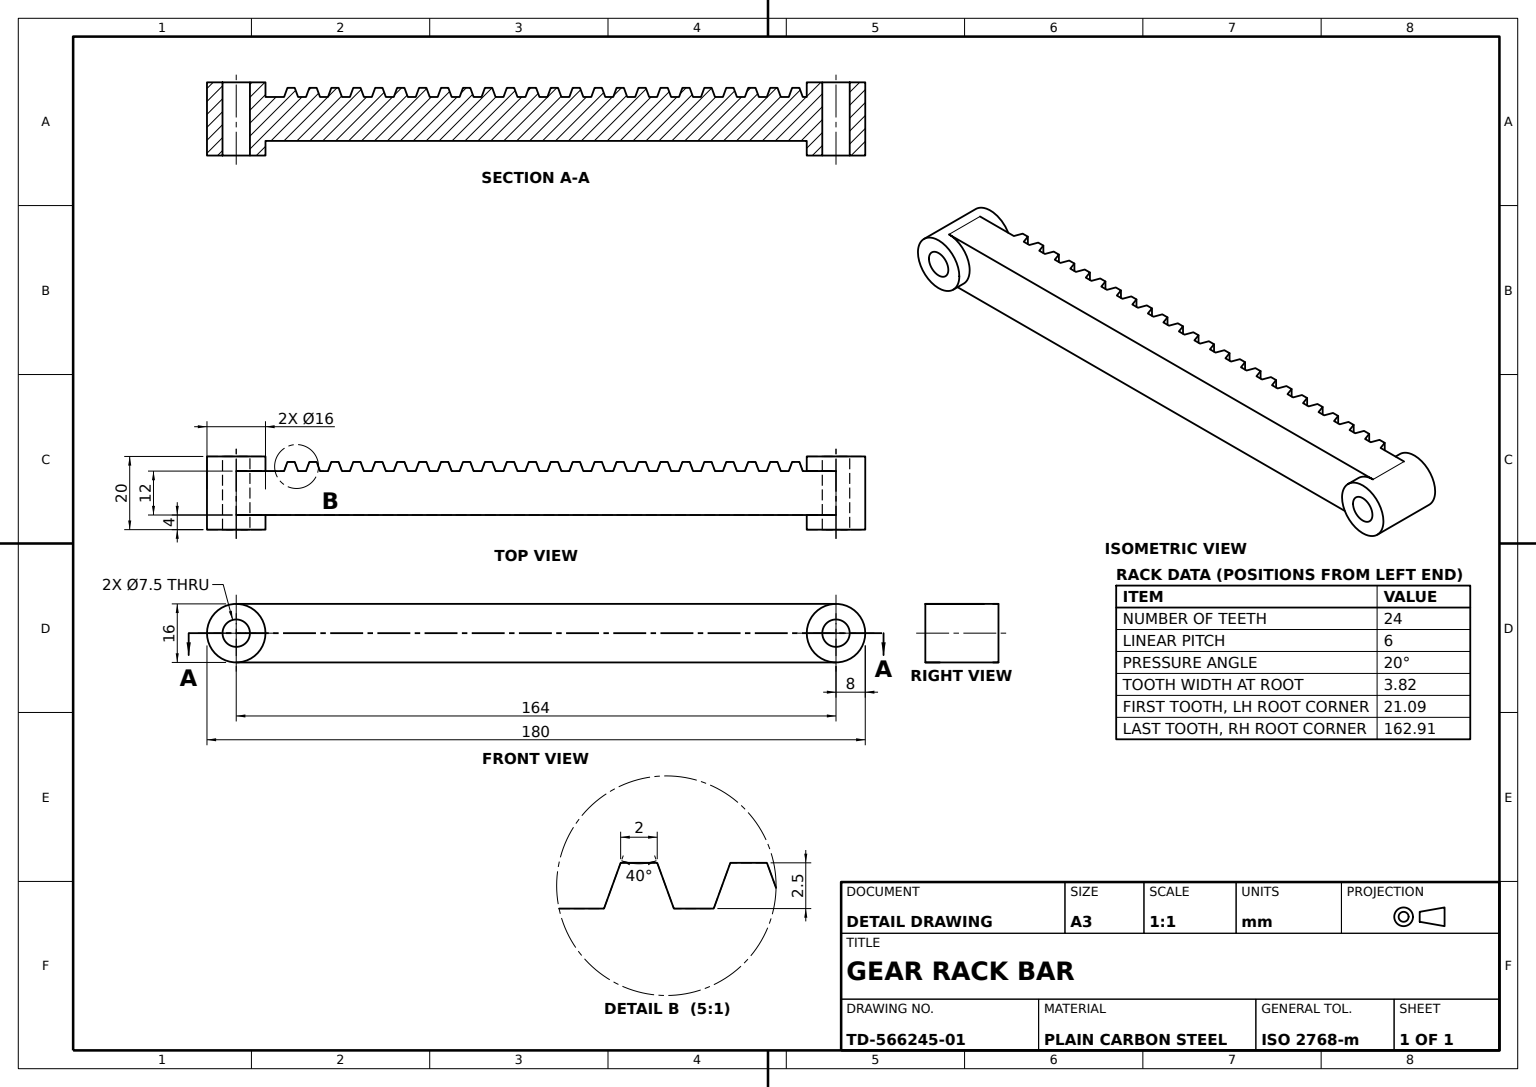
solid
v1 (10,0,8)
v2 (10,0,-8)
e1 v1 v2 CIRCLE(AX(P(10,0,0),D(1,0,0),D(0,0,-1)),8)
v3 (6,0,8)
e2 v1 v3 LINE
v4 (6,-8,0)
e3 v4 v3 CIRCLE(AX(P(6,0,0),D(-1,0,0),D(0,0,-1)),8)
v5 (-6,-8,0)
e4 v4 v5 LINE
v6 (-6,0,8)
e5 v5 v6 CIRCLE(AX(P(-6,0,0),D(-1,0,0),D(0,0,-1)),8)
v7 (-10,0,8)
e6 v6 v7 LINE
v8 (-10,0,-8)
e7 v7 v8 CIRCLE(AX(P(-10,0,0),D(1,0,0),D(0,0,-1)),8)
e8 v2 v8 LINE
face CYL(AX(P(10,0,0),D(-1,0,0),D(0,0,1)),8) [-e1 e2 -e3 e4 e5 e6 e7 -e8]
v9 (-8.5,8,100)
v10 (-8.5,8,102)
e9 v9 v10 LINE
v11 (-8.5,-8,100)
e10 v9 v11 LINE
v12 (-8.5,-8,102)
e11 v11 v12 LINE
e12 v10 v12 LINE
face PLANE(AX(P(-8.5,8,100),D(1,0,0),D(0,0,-1))) rev [-e9 e10 e11 -e12]
v13 (-6,-8,15.090074)
v14 (-6,-8,12.909926)
e13 v13 v14 LINE
v15 (-6,8,15.090074)
e14 v15 v13 LINE
v16 (-6,8,12.909926)
e15 v16 v15 LINE
e16 v14 v16 LINE
face PLANE(AX(P(-6,0,164),D(1,0,0),D(0,0,-1))) rev [-e13 -e14 -e15 -e16]
v17 (10,0,3.75)
v18 (-10,0,3.75)
e17 v17 v18 LINE
v19 (10,0,-3.75)
e18 v17 v19 CIRCLE(AX(P(10,0,0),D(1,0,0),D(0,0,-1)),3.75)
v20 (-10,0,-3.75)
e19 v19 v20 LINE
e20 v18 v20 CIRCLE(AX(P(-10,0,0),D(1,0,0),D(0,0,-1)),3.75)
face CYL(AX(P(10,0,0),D(-1,0,0),D(0,0,1)),3.75) rev [-e17 e18 e19 -e20]
v21 (-8.5,8,138)
v22 (-6,8,138.909926)
e21 v21 v22 LINE
v23 (-8.5,-8,138)
e22 v21 v23 LINE
v24 (-6,-8,138.909926)
e23 v23 v24 LINE
e24 v24 v22 LINE
face PLANE(AX(P(-8.5,8,138),D(0.342020143,0,-0.939692621),D(-0.939692621,0,-0.342020143))) rev [-e21 e22 e23 e24]
v25 (-6,8,27.090074)
v26 (-8.5,8,28)
e25 v25 v26 LINE
v27 (-6,-8,27.090074)
e26 v25 v27 LINE
v28 (-8.5,-8,28)
e27 v27 v28 LINE
e28 v26 v28 LINE
face PLANE(AX(P(-8.5,8,28),D(0.342020143,0,0.939692621),D(0.939692621,0,-0.342020143))) rev [-e25 e26 e27 -e28]
v29 (-8.5,8,36)
v30 (-6,8,36.909926)
e29 v29 v30 LINE
v31 (-8.5,-8,36)
e30 v29 v31 LINE
v32 (-6,-8,36.909926)
e31 v31 v32 LINE
e32 v32 v30 LINE
face PLANE(AX(P(-8.5,8,36),D(0.342020143,0,-0.939692621),D(-0.939692621,0,-0.342020143))) rev [-e29 e30 e31 e32]
v33 (-6,0,156)
v34 (-10,0,156)
e33 v33 v34 LINE
v35 (-10,0,172)
e34 v34 v35 CIRCLE(AX(P(-10,0,164),D(1,0,0),D(0,0,-1)),8)
v36 (10,0,172)
e35 v36 v35 LINE
v37 (10,0,156)
e36 v37 v36 CIRCLE(AX(P(10,0,164),D(1,0,0),D(0,0,-1)),8)
v38 (6,0,156)
e37 v37 v38 LINE
v39 (6,8,164)
e38 v39 v38 CIRCLE(AX(P(6,0,164),D(-1,0,0),D(0,0,-1)),8)
v40 (-6,8,164)
e39 v39 v40 LINE
e40 v40 v33 CIRCLE(AX(P(-6,0,164),D(-1,0,0),D(0,0,-1)),8)
face CYL(AX(P(10,0,164),D(-1,0,0),D(0,0,1)),8) [e33 e34 -e35 -e36 e37 -e38 e39 e40]
v41 (-8.5,8,124)
v42 (-8.5,8,126)
e41 v41 v42 LINE
v43 (-6,8,126.909926)
e42 v42 v43 LINE
v44 (-6,8,129.090074)
e43 v43 v44 LINE
v45 (-8.5,8,130)
e44 v44 v45 LINE
v46 (-8.5,8,132)
e45 v45 v46 LINE
v47 (-6,8,132.909926)
e46 v46 v47 LINE
v48 (-6,8,135.090074)
e47 v47 v48 LINE
v49 (-8.5,8,136)
e48 v48 v49 LINE
e49 v49 v21 LINE
v50 (-6,8,141.090074)
e50 v22 v50 LINE
v51 (-8.5,8,142)
e51 v50 v51 LINE
v52 (-8.5,8,144)
e52 v51 v52 LINE
v53 (-6,8,144.909926)
e53 v52 v53 LINE
v54 (-6,8,147.090074)
e54 v53 v54 LINE
v55 (-8.5,8,148)
e55 v54 v55 LINE
v56 (-8.5,8,150)
e56 v55 v56 LINE
v57 (-6,8,150.909926)
e57 v56 v57 LINE
e58 v57 v40 LINE
v58 (6,8,0)
e59 v58 v39 LINE
v59 (-6,8,0)
e60 v58 v59 LINE
v60 (-6,8,9.090074)
e61 v59 v60 LINE
v61 (-8.5,8,10)
e62 v60 v61 LINE
v62 (-8.5,8,12)
e63 v61 v62 LINE
e64 v62 v16 LINE
v63 (-8.5,8,16)
e65 v15 v63 LINE
v64 (-8.5,8,18)
e66 v63 v64 LINE
v65 (-6,8,18.909926)
e67 v64 v65 LINE
v66 (-6,8,21.090074)
e68 v65 v66 LINE
v67 (-8.5,8,22)
e69 v66 v67 LINE
v68 (-8.5,8,24)
e70 v67 v68 LINE
v69 (-6,8,24.909926)
e71 v68 v69 LINE
e72 v69 v25 LINE
v70 (-8.5,8,30)
e73 v26 v70 LINE
v71 (-6,8,30.909926)
e74 v70 v71 LINE
v72 (-6,8,33.090074)
e75 v71 v72 LINE
v73 (-8.5,8,34)
e76 v72 v73 LINE
e77 v73 v29 LINE
v74 (-6,8,39.090074)
e78 v30 v74 LINE
v75 (-8.5,8,40)
e79 v74 v75 LINE
v76 (-8.5,8,42)
e80 v75 v76 LINE
v77 (-6,8,42.909926)
e81 v76 v77 LINE
v78 (-6,8,45.090074)
e82 v77 v78 LINE
v79 (-8.5,8,46)
e83 v78 v79 LINE
v80 (-8.5,8,48)
e84 v79 v80 LINE
v81 (-6,8,48.909926)
e85 v80 v81 LINE
v82 (-6,8,51.090074)
e86 v81 v82 LINE
v83 (-8.5,8,52)
e87 v82 v83 LINE
v84 (-8.5,8,54)
e88 v83 v84 LINE
v85 (-6,8,54.909926)
e89 v84 v85 LINE
v86 (-6,8,57.090074)
e90 v85 v86 LINE
v87 (-8.5,8,58)
e91 v86 v87 LINE
v88 (-8.5,8,60)
e92 v87 v88 LINE
v89 (-6,8,60.909926)
e93 v88 v89 LINE
v90 (-6,8,63.090074)
e94 v89 v90 LINE
v91 (-8.5,8,64)
e95 v90 v91 LINE
v92 (-8.5,8,66)
e96 v91 v92 LINE
v93 (-6,8,66.909926)
e97 v92 v93 LINE
v94 (-6,8,69.090074)
e98 v93 v94 LINE
v95 (-8.5,8,70)
e99 v94 v95 LINE
v96 (-8.5,8,72)
e100 v95 v96 LINE
v97 (-6,8,72.909926)
e101 v96 v97 LINE
v98 (-6,8,75.090074)
e102 v97 v98 LINE
v99 (-8.5,8,76)
e103 v98 v99 LINE
v100 (-8.5,8,78)
e104 v99 v100 LINE
v101 (-6,8,78.909926)
e105 v100 v101 LINE
v102 (-6,8,81.090074)
e106 v101 v102 LINE
v103 (-8.5,8,82)
e107 v102 v103 LINE
v104 (-8.5,8,84)
e108 v103 v104 LINE
v105 (-6,8,84.909926)
e109 v104 v105 LINE
v106 (-6,8,87.090074)
e110 v105 v106 LINE
v107 (-8.5,8,88)
e111 v106 v107 LINE
v108 (-8.5,8,90)
e112 v107 v108 LINE
v109 (-6,8,90.909926)
e113 v108 v109 LINE
v110 (-6,8,93.090074)
e114 v109 v110 LINE
v111 (-8.5,8,94)
e115 v110 v111 LINE
v112 (-8.5,8,96)
e116 v111 v112 LINE
v113 (-6,8,96.909926)
e117 v112 v113 LINE
v114 (-6,8,99.090074)
e118 v113 v114 LINE
e119 v114 v9 LINE
v115 (-6,8,102.909926)
e120 v10 v115 LINE
v116 (-6,8,105.090074)
e121 v115 v116 LINE
v117 (-8.5,8,106)
e122 v116 v117 LINE
v118 (-8.5,8,108)
e123 v117 v118 LINE
v119 (-6,8,108.909926)
e124 v118 v119 LINE
v120 (-6,8,111.090074)
e125 v119 v120 LINE
v121 (-8.5,8,112)
e126 v120 v121 LINE
v122 (-8.5,8,114)
e127 v121 v122 LINE
v123 (-6,8,114.909926)
e128 v122 v123 LINE
v124 (-6,8,117.090074)
e129 v123 v124 LINE
v125 (-8.5,8,118)
e130 v124 v125 LINE
v126 (-8.5,8,120)
e131 v125 v126 LINE
v127 (-6,8,120.909926)
e132 v126 v127 LINE
v128 (-6,8,123.090074)
e133 v127 v128 LINE
e134 v128 v41 LINE
face PLANE(AX(P(6,8,164),D(0,-1,0),D(0,0,-1))) rev [e41 e42 e43 e44 e45 e46 e47 e48 e49 e21 e50 e51 e52 e53 e54 e55 e56 e57 e58 -e39 -e59 e60 e61 e62 e63 e64 e15 e65 e66 e67 e68 e69 e70 e71 e72 e25 e73 e74 e75 e76 e77 e29 e78 e79 e80 e81 e82 e83 e84 e85 e86 e87 e88 e89 e90 e91 e92 e93 e94 e95 e96 e97 e98 e99 e100 e101 e102 e103 e104 e105 e106 e107 e108 e109 e110 e111 e112 e113 e114 e115 e116 e117 e118 e119 e9 e120 e121 e122 e123 e124 e125 e126 e127 e128 e129 e130 e131 e132 e133 e134]
v129 (-6,-8,21.090074)
v130 (-8.5,-8,22)
e135 v129 v130 LINE
e136 v67 v130 LINE
e137 v66 v129 LINE
face PLANE(AX(P(-8.5,8,22),D(0.342020143,0,0.939692621),D(0.939692621,0,-0.342020143))) rev [e135 -e136 -e69 e137]
v131 (-8.5,-8,70)
e138 v95 v131 LINE
v132 (-8.5,-8,72)
e139 v131 v132 LINE
e140 v96 v132 LINE
face PLANE(AX(P(-8.5,8,70),D(1,0,0),D(0,0,-1))) rev [e138 e139 -e140 -e100]
v133 (-8.5,-8,24)
e141 v130 v133 LINE
e142 v68 v133 LINE
face PLANE(AX(P(-8.5,8,22),D(1,0,0),D(0,0,-1))) rev [-e70 e136 e141 -e142]
v134 (-6,-8,99.090074)
v135 (-6,-8,96.909926)
e143 v134 v135 LINE
e144 v114 v134 LINE
e145 v135 v113 LINE
face PLANE(AX(P(-6,0,164),D(1,0,0),D(0,0,-1))) rev [-e143 -e144 -e118 -e145]
v136 (-6,-8,69.090074)
e146 v136 v131 LINE
v137 (-6,-8,66.909926)
e147 v136 v137 LINE
v138 (-8.5,-8,66)
e148 v138 v137 LINE
v139 (-8.5,-8,64)
e149 v139 v138 LINE
v140 (-6,-8,63.090074)
e150 v140 v139 LINE
v141 (-6,-8,60.909926)
e151 v140 v141 LINE
v142 (-8.5,-8,60)
e152 v142 v141 LINE
v143 (-8.5,-8,58)
e153 v143 v142 LINE
v144 (-6,-8,57.090074)
e154 v144 v143 LINE
v145 (-6,-8,54.909926)
e155 v144 v145 LINE
v146 (-8.5,-8,54)
e156 v146 v145 LINE
v147 (-8.5,-8,52)
e157 v147 v146 LINE
v148 (-6,-8,51.090074)
e158 v148 v147 LINE
v149 (-6,-8,48.909926)
e159 v148 v149 LINE
v150 (-8.5,-8,48)
e160 v150 v149 LINE
v151 (-8.5,-8,46)
e161 v151 v150 LINE
v152 (-6,-8,45.090074)
e162 v152 v151 LINE
v153 (-6,-8,42.909926)
e163 v152 v153 LINE
v154 (-8.5,-8,42)
e164 v154 v153 LINE
v155 (-8.5,-8,40)
e165 v155 v154 LINE
v156 (-6,-8,39.090074)
e166 v156 v155 LINE
e167 v156 v32 LINE
v157 (-8.5,-8,34)
e168 v157 v31 LINE
v158 (-6,-8,33.090074)
e169 v158 v157 LINE
v159 (-6,-8,30.909926)
e170 v158 v159 LINE
v160 (-8.5,-8,30)
e171 v160 v159 LINE
e172 v28 v160 LINE
v161 (-6,-8,24.909926)
e173 v27 v161 LINE
e174 v133 v161 LINE
v162 (-6,-8,18.909926)
e175 v129 v162 LINE
v163 (-8.5,-8,18)
e176 v163 v162 LINE
v164 (-8.5,-8,16)
e177 v164 v163 LINE
e178 v13 v164 LINE
v165 (-8.5,-8,12)
e179 v165 v14 LINE
v166 (-8.5,-8,10)
e180 v166 v165 LINE
v167 (-6,-8,9.090074)
e181 v167 v166 LINE
e182 v167 v5 LINE
v168 (6,-8,164)
e183 v168 v4 LINE
v169 (-6,-8,164)
e184 v168 v169 LINE
v170 (-6,-8,150.909926)
e185 v169 v170 LINE
v171 (-8.5,-8,150)
e186 v171 v170 LINE
v172 (-8.5,-8,148)
e187 v172 v171 LINE
v173 (-6,-8,147.090074)
e188 v173 v172 LINE
v174 (-6,-8,144.909926)
e189 v173 v174 LINE
v175 (-8.5,-8,144)
e190 v175 v174 LINE
v176 (-8.5,-8,142)
e191 v176 v175 LINE
v177 (-6,-8,141.090074)
e192 v177 v176 LINE
e193 v177 v24 LINE
v178 (-8.5,-8,136)
e194 v178 v23 LINE
v179 (-6,-8,135.090074)
e195 v179 v178 LINE
v180 (-6,-8,132.909926)
e196 v179 v180 LINE
v181 (-8.5,-8,132)
e197 v181 v180 LINE
v182 (-8.5,-8,130)
e198 v182 v181 LINE
v183 (-6,-8,129.090074)
e199 v183 v182 LINE
v184 (-6,-8,126.909926)
e200 v183 v184 LINE
v185 (-8.5,-8,126)
e201 v185 v184 LINE
v186 (-8.5,-8,124)
e202 v186 v185 LINE
v187 (-6,-8,123.090074)
e203 v187 v186 LINE
v188 (-6,-8,120.909926)
e204 v187 v188 LINE
v189 (-8.5,-8,120)
e205 v189 v188 LINE
v190 (-8.5,-8,118)
e206 v190 v189 LINE
v191 (-6,-8,117.090074)
e207 v191 v190 LINE
v192 (-6,-8,114.909926)
e208 v191 v192 LINE
v193 (-8.5,-8,114)
e209 v193 v192 LINE
v194 (-8.5,-8,112)
e210 v194 v193 LINE
v195 (-6,-8,111.090074)
e211 v195 v194 LINE
v196 (-6,-8,108.909926)
e212 v195 v196 LINE
v197 (-8.5,-8,108)
e213 v197 v196 LINE
v198 (-8.5,-8,106)
e214 v198 v197 LINE
v199 (-6,-8,105.090074)
e215 v199 v198 LINE
v200 (-6,-8,102.909926)
e216 v199 v200 LINE
e217 v12 v200 LINE
e218 v134 v11 LINE
v201 (-8.5,-8,96)
e219 v201 v135 LINE
v202 (-8.5,-8,94)
e220 v202 v201 LINE
v203 (-6,-8,93.090074)
e221 v203 v202 LINE
v204 (-6,-8,90.909926)
e222 v203 v204 LINE
v205 (-8.5,-8,90)
e223 v205 v204 LINE
v206 (-8.5,-8,88)
e224 v206 v205 LINE
v207 (-6,-8,87.090074)
e225 v207 v206 LINE
v208 (-6,-8,84.909926)
e226 v207 v208 LINE
v209 (-8.5,-8,84)
e227 v209 v208 LINE
v210 (-8.5,-8,82)
e228 v210 v209 LINE
v211 (-6,-8,81.090074)
e229 v211 v210 LINE
v212 (-6,-8,78.909926)
e230 v211 v212 LINE
v213 (-8.5,-8,78)
e231 v213 v212 LINE
v214 (-8.5,-8,76)
e232 v214 v213 LINE
v215 (-6,-8,75.090074)
e233 v215 v214 LINE
v216 (-6,-8,72.909926)
e234 v215 v216 LINE
e235 v132 v216 LINE
face PLANE(AX(P(6,-8,164),D(0,1,0),D(0,0,1))) rev [-e139 -e146 e147 -e148 -e149 -e150 e151 -e152 -e153 -e154 e155 -e156 -e157 -e158 e159 -e160 -e161 -e162 e163 -e164 -e165 -e166 e167 -e31 -e168 -e169 e170 -e171 -e172 -e27 e173 -e174 -e141 -e135 e175 -e176 -e177 -e178 e13 -e179 -e180 -e181 e182 -e4 -e183 e184 e185 -e186 -e187 -e188 e189 -e190 -e191 -e192 e193 -e23 -e194 -e195 e196 -e197 -e198 -e199 e200 -e201 -e202 -e203 e204 -e205 -e206 -e207 e208 -e209 -e210 -e211 e212 -e213 -e214 -e215 e216 -e217 -e11 -e218 e143 -e219 -e220 -e221 e222 -e223 -e224 -e225 e226 -e227 -e228 -e229 e230 -e231 -e232 -e233 e234 -e235]
e236 v56 v171 LINE
e237 v170 v57 LINE
face PLANE(AX(P(-8.5,8,150),D(0.342020143,0,-0.939692621),D(-0.939692621,0,-0.342020143))) rev [e236 e186 e237 -e57]
e238 v62 v165 LINE
face PLANE(AX(P(-8.5,8,12),D(0.342020143,0,-0.939692621),D(-0.939692621,0,-0.342020143))) rev [e16 -e64 e238 e179]
e239 v91 v139 LINE
e240 v92 v138 LINE
face PLANE(AX(P(-8.5,8,64),D(1,0,0),D(0,0,-1))) rev [-e96 e239 e149 -e240]
e241 v74 v156 LINE
face PLANE(AX(P(-6,0,164),D(1,0,0),D(0,0,-1))) rev [-e78 -e32 -e167 -e241]
e242 v19 v17 CIRCLE(AX(P(10,0,0),D(1,0,0),D(0,0,-1)),3.75)
e243 v20 v18 CIRCLE(AX(P(-10,0,0),D(1,0,0),D(0,0,-1)),3.75)
face CYL(AX(P(10,0,0),D(-1,0,0),D(0,0,1)),3.75) rev [-e19 e242 e17 -e243]
e244 v55 v172 LINE
face PLANE(AX(P(-8.5,8,148),D(1,0,0),D(0,0,-1))) rev [e187 -e236 -e56 e244]
e245 v196 v119 LINE
e246 v118 v197 LINE
face PLANE(AX(P(-8.5,8,108),D(0.342020143,0,-0.939692621),D(-0.939692621,0,-0.342020143))) rev [e213 e245 -e124 e246]
e247 v200 v115 LINE
e248 v116 v199 LINE
face PLANE(AX(P(-6,0,164),D(1,0,0),D(0,0,-1))) rev [-e247 -e216 -e248 -e121]
e249 v108 v205 LINE
e250 v204 v109 LINE
face PLANE(AX(P(-8.5,8,90),D(0.342020143,0,-0.939692621),D(-0.939692621,0,-0.342020143))) rev [e249 e223 e250 -e113]
e251 v86 v144 LINE
e252 v87 v143 LINE
face PLANE(AX(P(-8.5,8,58),D(0.342020143,0,0.939692621),D(0.939692621,0,-0.342020143))) rev [-e91 e251 e154 -e252]
e253 v8 v7 CIRCLE(AX(P(-10,0,0),D(1,0,0),D(0,0,-1)),8)
e254 v6 v59 CIRCLE(AX(P(-6,0,0),D(-1,0,0),D(0,0,-1)),8)
e255 v3 v58 CIRCLE(AX(P(6,0,0),D(-1,0,0),D(0,0,-1)),8)
e256 v2 v1 CIRCLE(AX(P(10,0,0),D(1,0,0),D(0,0,-1)),8)
face CYL(AX(P(10,0,0),D(-1,0,0),D(0,0,1)),8) [e8 e253 -e6 e254 -e60 -e255 -e2 -e256]
e257 v94 v136 LINE
face PLANE(AX(P(-8.5,8,70),D(0.342020143,0,0.939692621),D(0.939692621,0,-0.342020143))) rev [-e138 -e99 e257 e146]
e258 v80 v150 LINE
e259 v149 v81 LINE
face PLANE(AX(P(-8.5,8,48),D(0.342020143,0,-0.939692621),D(-0.939692621,0,-0.342020143))) rev [-e85 e258 e160 e259]
e260 v184 v43 LINE
e261 v42 v185 LINE
face PLANE(AX(P(-8.5,8,126),D(0.342020143,0,-0.939692621),D(-0.939692621,0,-0.342020143))) rev [e260 -e42 e261 e201]
e262 v51 v176 LINE
e263 v52 v175 LINE
face PLANE(AX(P(-8.5,8,142),D(1,0,0),D(0,0,-1))) rev [e262 e191 -e263 -e52]
e264 v45 v182 LINE
e265 v44 v183 LINE
face PLANE(AX(P(-8.5,8,130),D(0.342020143,0,0.939692621),D(0.939692621,0,-0.342020143))) rev [-e264 -e44 e265 e199]
e266 v112 v201 LINE
face PLANE(AX(P(-8.5,8,96),D(0.342020143,0,-0.939692621),D(-0.939692621,0,-0.342020143))) rev [e266 e219 e145 -e117]
e267 v128 v187 LINE
e268 v41 v186 LINE
face PLANE(AX(P(-8.5,8,124),D(0.342020143,0,0.939692621),D(0.939692621,0,-0.342020143))) rev [-e134 e267 e203 -e268]
e269 v117 v198 LINE
face PLANE(AX(P(-8.5,8,106),D(0.342020143,0,0.939692621),D(0.939692621,0,-0.342020143))) rev [e248 e215 -e269 -e122]
face PLANE(AX(P(-8.5,8,124),D(1,0,0),D(0,0,-1))) rev [-e41 e268 e202 -e261]
e270 v98 v215 LINE
e271 v99 v214 LINE
face PLANE(AX(P(-8.5,8,76),D(0.342020143,0,0.939692621),D(0.939692621,0,-0.342020143))) rev [-e103 e270 e233 -e271]
e272 v188 v127 LINE
face PLANE(AX(P(-6,0,164),D(1,0,0),D(0,0,-1))) rev [-e133 -e272 -e204 -e267]
e273 v100 v213 LINE
face PLANE(AX(P(-8.5,8,76),D(1,0,0),D(0,0,-1))) rev [-e104 e271 e232 -e273]
e274 v64 v163 LINE
e275 v162 v65 LINE
face PLANE(AX(P(-8.5,8,18),D(0.342020143,0,-0.939692621),D(-0.939692621,0,-0.342020143))) rev [-e67 e274 e176 e275]
e276 v35 v34 CIRCLE(AX(P(-10,0,164),D(1,0,0),D(0,0,-1)),8)
e277 v33 v169 CIRCLE(AX(P(-6,0,164),D(-1,0,0),D(0,0,-1)),8)
e278 v38 v168 CIRCLE(AX(P(6,0,164),D(-1,0,0),D(0,0,-1)),8)
e279 v36 v37 CIRCLE(AX(P(10,0,164),D(1,0,0),D(0,0,-1)),8)
face CYL(AX(P(10,0,164),D(-1,0,0),D(0,0,1)),8) [e35 e276 -e33 e277 -e184 -e278 -e37 -e279]
e280 v174 v53 LINE
face PLANE(AX(P(-8.5,8,144),D(0.342020143,0,-0.939692621),D(-0.939692621,0,-0.342020143))) rev [e263 e190 e280 -e53]
e281 v106 v207 LINE
e282 v208 v105 LINE
face PLANE(AX(P(-6,0,164),D(1,0,0),D(0,0,-1))) rev [-e281 -e110 -e282 -e226]
face PLANE(AX(P(10,0,0),D(1,0,0),D(0,0,-1))) [e1 e256] [-e242 -e18]
e283 v72 v158 LINE
e284 v73 v157 LINE
face PLANE(AX(P(-8.5,8,34),D(0.342020143,0,0.939692621),D(0.939692621,0,-0.342020143))) rev [-e76 e283 e169 -e284]
e285 v192 v123 LINE
e286 v122 v193 LINE
face PLANE(AX(P(-8.5,8,114),D(0.342020143,0,-0.939692621),D(-0.939692621,0,-0.342020143))) rev [e209 e285 -e128 e286]
e287 v103 v210 LINE
e288 v104 v209 LINE
face PLANE(AX(P(-8.5,8,82),D(1,0,0),D(0,0,-1))) rev [-e108 e287 e228 -e288]
e289 v107 v206 LINE
face PLANE(AX(P(-8.5,8,88),D(0.342020143,0,0.939692621),D(0.939692621,0,-0.342020143))) rev [-e111 e281 e225 -e289]
e290 v83 v147 LINE
e291 v84 v146 LINE
face PLANE(AX(P(-8.5,8,52),D(1,0,0),D(0,0,-1))) rev [e290 e157 -e291 -e88]
face PLANE(AX(P(-6,0,164),D(1,0,0),D(0,0,-1))) rev [-e260 -e200 -e265 -e43]
e292 v161 v69 LINE
face PLANE(AX(P(-6,0,164),D(1,0,0),D(0,0,-1))) rev [-e26 -e72 -e292 -e173]
e293 v78 v152 LINE
e294 v153 v77 LINE
face PLANE(AX(P(-6,0,164),D(1,0,0),D(0,0,-1))) rev [-e293 -e82 -e294 -e163]
e295 v121 v194 LINE
face PLANE(AX(P(-8.5,8,112),D(1,0,0),D(0,0,-1))) rev [e210 -e286 -e127 e295]
e296 v110 v203 LINE
e297 v111 v202 LINE
face PLANE(AX(P(-8.5,8,94),D(0.342020143,0,0.939692621),D(0.939692621,0,-0.342020143))) rev [-e115 e296 e221 -e297]
e298 v76 v154 LINE
face PLANE(AX(P(-8.5,8,42),D(0.342020143,0,-0.939692621),D(-0.939692621,0,-0.342020143))) rev [e294 -e81 e298 e164]
face PLANE(AX(P(-6,0,164),D(1,0,0),D(0,0,-1))) rev [-e275 -e175 -e137 -e68]
e299 v141 v89 LINE
e300 v90 v140 LINE
face PLANE(AX(P(-6,0,164),D(1,0,0),D(0,0,-1))) rev [-e94 -e299 -e151 -e300]
v217 (10,0,160.25)
v218 (-10,0,160.25)
e301 v217 v218 LINE
v219 (10,0,167.75)
e302 v217 v219 CIRCLE(AX(P(10,0,164),D(1,0,0),D(0,0,-1)),3.75)
v220 (-10,0,167.75)
e303 v219 v220 LINE
e304 v218 v220 CIRCLE(AX(P(-10,0,164),D(1,0,0),D(0,0,-1)),3.75)
face CYL(AX(P(10,0,164),D(-1,0,0),D(0,0,1)),3.75) rev [-e301 e302 e303 -e304]
face PLANE(AX(P(-8.5,8,100),D(0.342020143,0,0.939692621),D(0.939692621,0,-0.342020143))) rev [-e119 e144 e218 -e10]
e305 v145 v85 LINE
face PLANE(AX(P(-8.5,8,54),D(0.342020143,0,-0.939692621),D(-0.939692621,0,-0.342020143))) rev [e291 e156 e305 -e89]
e306 v75 v155 LINE
face PLANE(AX(P(-8.5,8,40),D(0.342020143,0,0.939692621),D(0.939692621,0,-0.342020143))) rev [-e306 -e79 e241 e166]
face PLANE(AX(P(-8.5,8,40),D(1,0,0),D(0,0,-1))) rev [e306 e165 -e298 -e80]
e307 v79 v151 LINE
face PLANE(AX(P(-8.5,8,46),D(0.342020143,0,0.939692621),D(0.939692621,0,-0.342020143))) rev [e293 e162 -e307 -e83]
face PLANE(AX(P(-8.5,8,46),D(1,0,0),D(0,0,-1))) rev [e307 e161 -e258 -e84]
e308 v220 v218 CIRCLE(AX(P(-10,0,164),D(1,0,0),D(0,0,-1)),3.75)
e309 v219 v217 CIRCLE(AX(P(10,0,164),D(1,0,0),D(0,0,-1)),3.75)
face CYL(AX(P(10,0,164),D(-1,0,0),D(0,0,1)),3.75) rev [e301 -e308 -e303 e309]
face PLANE(AX(P(-8.5,8,24),D(0.342020143,0,-0.939692621),D(-0.939692621,0,-0.342020143))) rev [e292 -e71 e142 e174]
e310 v102 v211 LINE
face PLANE(AX(P(-8.5,8,82),D(0.342020143,0,0.939692621),D(0.939692621,0,-0.342020143))) rev [-e107 e310 e229 -e287]
face PLANE(AX(P(-8.5,8,102),D(0.342020143,0,-0.939692621),D(-0.939692621,0,-0.342020143))) rev [-e120 e12 e217 e247]
e311 v63 v164 LINE
face PLANE(AX(P(-8.5,8,16),D(0.342020143,0,0.939692621),D(0.939692621,0,-0.342020143))) rev [e14 e178 -e311 -e65]
e312 v46 v181 LINE
e313 v180 v47 LINE
face PLANE(AX(P(-8.5,8,132),D(0.342020143,0,-0.939692621),D(-0.939692621,0,-0.342020143))) rev [e312 e197 e313 -e46]
e314 v88 v142 LINE
face PLANE(AX(P(-8.5,8,60),D(0.342020143,0,-0.939692621),D(-0.939692621,0,-0.342020143))) rev [e152 e299 -e93 e314]
e315 v82 v148 LINE
face PLANE(AX(P(-6,0,164),D(1,0,0),D(0,0,-1))) rev [-e86 -e259 -e159 -e315]
face PLANE(AX(P(-10,0,0),D(1,0,0),D(0,0,-1))) rev [-e253 -e7] [e20 e243]
e316 v70 v160 LINE
face PLANE(AX(P(-8.5,8,28),D(1,0,0),D(0,0,-1))) rev [e28 e172 -e316 -e73]
face PLANE(AX(P(10,0,164),D(1,0,0),D(0,0,-1))) [e36 e279] [-e309 -e302]
face PLANE(AX(P(-6,0,164),D(1,0,0),D(0,0,-1))) rev [-e40 -e58 -e237 -e185 -e277]
e317 v126 v189 LINE
face PLANE(AX(P(-8.5,8,120),D(0.342020143,0,-0.939692621),D(-0.939692621,0,-0.342020143))) rev [-e132 e317 e205 e272]
e318 v49 v178 LINE
face PLANE(AX(P(-8.5,8,136),D(1,0,0),D(0,0,-1))) rev [-e49 e318 e194 -e22]
e319 v159 v71 LINE
face PLANE(AX(P(-8.5,8,30),D(0.342020143,0,-0.939692621),D(-0.939692621,0,-0.342020143))) rev [e171 e319 -e74 e316]
e320 v120 v195 LINE
face PLANE(AX(P(-8.5,8,112),D(0.342020143,0,0.939692621),D(0.939692621,0,-0.342020143))) rev [-e126 e320 e211 -e295]
e321 v50 v177 LINE
face PLANE(AX(P(-8.5,8,142),D(0.342020143,0,0.939692621),D(0.939692621,0,-0.342020143))) rev [e321 e192 -e262 -e51]
face PLANE(AX(P(6,0,164),D(1,0,0),D(0,0,-1))) [e59 e38 e278 e183 e3 e255]
face PLANE(AX(P(-8.5,8,88),D(1,0,0),D(0,0,-1))) rev [-e112 e289 e224 -e249]
face PLANE(AX(P(-6,0,164),D(1,0,0),D(0,0,-1))) rev [-e319 -e170 -e283 -e75]
face PLANE(AX(P(-8.5,8,106),D(1,0,0),D(0,0,-1))) rev [e269 e214 -e246 -e123]
face PLANE(AX(P(-8.5,8,84),D(0.342020143,0,-0.939692621),D(-0.939692621,0,-0.342020143))) rev [e227 e282 -e109 e288]
e322 v60 v167 LINE
face PLANE(AX(P(-6,0,164),D(1,0,0),D(0,0,-1))) rev [-e182 -e322 -e61 -e254 -e5]
e323 v125 v190 LINE
e324 v124 v191 LINE
face PLANE(AX(P(-8.5,8,118),D(0.342020143,0,0.939692621),D(0.939692621,0,-0.342020143))) rev [-e323 -e130 e324 e207]
e325 v137 v93 LINE
face PLANE(AX(P(-8.5,8,66),D(0.342020143,0,-0.939692621),D(-0.939692621,0,-0.342020143))) rev [e325 -e97 e240 e148]
face PLANE(AX(P(-8.5,8,52),D(0.342020143,0,0.939692621),D(0.939692621,0,-0.342020143))) rev [-e87 e315 e158 -e290]
face PLANE(AX(P(-8.5,8,64),D(0.342020143,0,0.939692621),D(0.939692621,0,-0.342020143))) rev [-e95 e300 e150 -e239]
face PLANE(AX(P(-6,0,164),D(1,0,0),D(0,0,-1))) rev [-e193 -e321 -e50 -e24]
face PLANE(AX(P(-6,0,164),D(1,0,0),D(0,0,-1))) rev [-e305 -e155 -e251 -e90]
face PLANE(AX(P(-6,0,164),D(1,0,0),D(0,0,-1))) rev [-e245 -e212 -e320 -e125]
face PLANE(AX(P(-8.5,8,118),D(1,0,0),D(0,0,-1))) rev [-e317 -e131 e323 e206]
e326 v61 v166 LINE
face PLANE(AX(P(-8.5,8,10),D(1,0,0),D(0,0,-1))) rev [-e63 e326 e180 -e238]
e327 v54 v173 LINE
face PLANE(AX(P(-8.5,8,148),D(0.342020143,0,0.939692621),D(0.939692621,0,-0.342020143))) rev [e327 e188 -e244 -e55]
face PLANE(AX(P(-6,0,164),D(1,0,0),D(0,0,-1))) rev [-e208 -e324 -e129 -e285]
face PLANE(AX(P(-6,0,164),D(1,0,0),D(0,0,-1))) rev [-e222 -e296 -e114 -e250]
face PLANE(AX(P(-8.5,8,58),D(1,0,0),D(0,0,-1))) rev [e153 -e314 -e92 e252]
e328 v212 v101 LINE
face PLANE(AX(P(-6,0,164),D(1,0,0),D(0,0,-1))) rev [-e310 -e106 -e328 -e230]
face PLANE(AX(P(-6,0,164),D(1,0,0),D(0,0,-1))) rev [-e327 -e54 -e280 -e189]
face PLANE(AX(P(-8.5,8,34),D(1,0,0),D(0,0,-1))) rev [e284 e168 -e30 -e77]
face PLANE(AX(P(-10,0,164),D(1,0,0),D(0,0,-1))) rev [-e276 -e34] [e308 e304]
face PLANE(AX(P(-8.5,8,78),D(0.342020143,0,-0.939692621),D(-0.939692621,0,-0.342020143))) rev [e273 e231 e328 -e105]
face PLANE(AX(P(-6,0,164),D(1,0,0),D(0,0,-1))) rev [-e98 -e325 -e147 -e257]
face PLANE(AX(P(-8.5,8,94),D(1,0,0),D(0,0,-1))) rev [e297 e220 -e266 -e116]
e329 v48 v179 LINE
face PLANE(AX(P(-6,0,164),D(1,0,0),D(0,0,-1))) rev [-e313 -e196 -e329 -e47]
e330 v216 v97 LINE
face PLANE(AX(P(-8.5,8,72),D(0.342020143,0,-0.939692621),D(-0.939692621,0,-0.342020143))) rev [e235 e330 -e101 e140]
face PLANE(AX(P(-8.5,8,130),D(1,0,0),D(0,0,-1))) rev [-e312 -e45 e264 e198]
face PLANE(AX(P(-6,0,164),D(1,0,0),D(0,0,-1))) rev [-e102 -e330 -e234 -e270]
face PLANE(AX(P(-8.5,8,16),D(1,0,0),D(0,0,-1))) rev [-e274 -e66 e311 e177]
face PLANE(AX(P(-8.5,8,10),D(0.342020143,0,0.939692621),D(0.939692621,0,-0.342020143))) rev [-e326 -e62 e322 e181]
face PLANE(AX(P(-8.5,8,136),D(0.342020143,0,0.939692621),D(0.939692621,0,-0.342020143))) rev [-e318 -e48 e329 e195]
